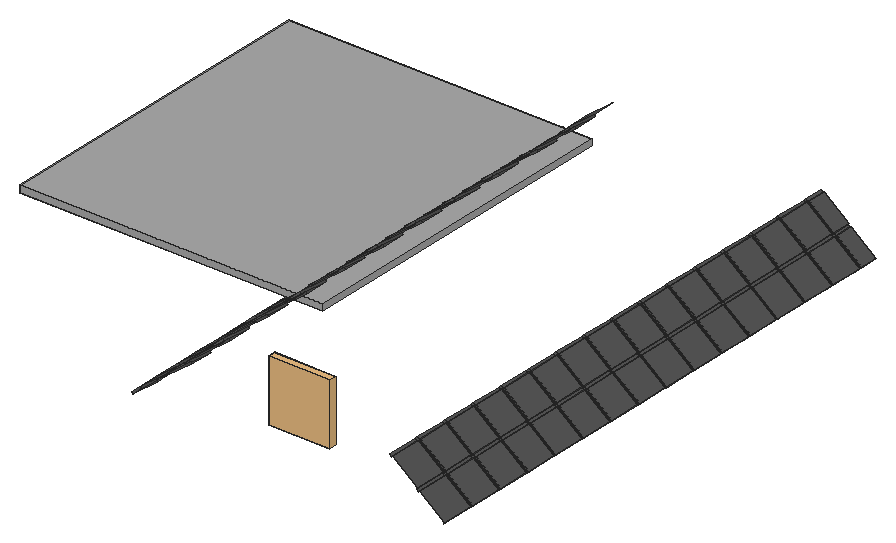
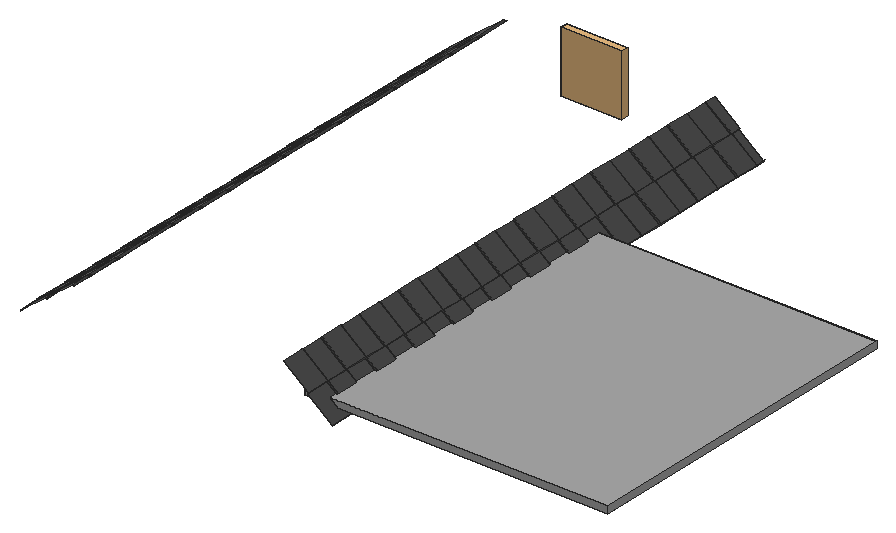
# SketchUp Ruby script. Lengths in inches.
U = 1.inch
M = Sketchup.active_model
def pt(a) = Geom::Point3d.new(a.map { |v| v * U })
def face(e, loops, mat)
  f = e.add_face(loops[0].map { |a| pt(a) })
  loops[1..].each { |l| e.add_face(l.map { |a| pt(a) }).erase! }
  f.material = f.back_material = mat if mat
  f
end
# faces: each face lists its corners as indices into pts; further lists are holes
def faces(e, pts, list, mat = nil) = list.each { |f| face(e, (f[0].is_a?(Array) ? f : [f]).map { |l| l.map { |i| pts[i] } }, mat) }
# xy, xz, yz: faces in a plane at the given z, y or x. An outline is a flat list of corners, or four numbers for a rectangle; further outlines are holes
def ring(l) = l.size == 4 ? [[l[0], l[1]], [l[2], l[1]], [l[2], l[3]], [l[0], l[3]]] : l.each_slice(2).to_a
def flat(e, list, mat, &to3) = list.each { |f| face(e, (f[0].is_a?(Array) ? f : [f]).map { |l| ring(l).map { |u, v| to3.(u, v) } }, mat) }
def xy(e, z, list, mat = nil) = flat(e, list, mat) { |x, y| [x, y, z] }
def xz(e, y, list, mat = nil) = flat(e, list, mat) { |x, z| [x, y, z] }
def yz(e, x, list, mat = nil) = flat(e, list, mat) { |y, z| [x, y, z] }
def lines(e, pts, list) = list.each { |a, b| e.add_line(pt(pts[a]), pt(pts[b])) }
# prism: a flat outline (further loops are holes) pulled along v
def prism(e, loops, v, mat = nil)
  f = face(e, loops, mat); d = Geom::Vector3d.new(v.map { |x| x * U })
  f.pushpull(f.normal.samedirection?(d) ? d.length : -d.length)
end
def box(e, o, s, mat = nil) = prism(e, [[o, [o[0] + s[0], o[1], o[2]], [o[0] + s[0], o[1] + s[1], o[2]], [o[0], o[1] + s[1], o[2]]]], [0, 0, s[2]], mat)
def at(x, y, z, deg = 0) = Geom::Transformation.translation(pt([x, y, z])) * Geom::Transformation.rotation(ORIGIN, Z_AXIS, deg.degrees)
def axes(o, x, y, z) = Geom::Transformation.new([*x, 0, *y, 0, *z, 0, *pt(o).to_a, 1])
def part(name) = M.definitions.add(name)
# library, detail: a bought-in or finely detailed component or shape, given as its bounding box
def library(name, o, s) = part(name).tap { |d| box(d.entities, o, s) }
def detail(e, o, s) = box(e.add_group.entities, o, s)
def put(e, d, t, mat = nil) = e.add_instance(d, t).tap { |i| i.material = mat if mat }
def group(e, t, mat = nil) = e.add_group.tap { |g| g.transformation = t; g.material = mat if mat }.entities
root = M.entities
M.materials.add("[Color M03]").color = [170, 170, 170]
M.materials.add("[Color M05]").color = [114, 114, 114]
M.materials.add("[Color M06]").color = [86, 86, 86]
c1 = library("Group\#78",[0,-0.5,0],[45.98,5.5,45.98])
xz(root,145.1875,[[263.93,349.38,282.83,364.17,282.34,364.8,282.03,365.19,263.13,350.4,263.4375,350.01],[282.83,364.17,282.34,364.8,282.03,365.19,300.93,379.98,301.24,379.59,301.73,378.96]],"[Color M06]")
xz(root,161.375,[[497.33,344.21,478.43,359.01,479.05,359.79,497.95,345],[476.86,360.24,457.95,375.03,458.57,375.82,477.47,361.03]],"[Color M06]")
xz(root,163.1875,[[263.93,349.38,263.4375,350.01,263.13,350.4,282.03,365.19,282.34,364.8,282.83,364.17],[282.83,364.17,301.73,378.96,301.24,379.59,300.93,379.98,282.03,365.19,282.34,364.8]],"[Color M06]")
xz(root,163.375,[[497.33,344.21,497.95,345,479.05,359.79,478.43,359.01],[476.86,360.24,477.47,361.03,458.57,375.82,457.95,375.03]],"[Color M06]")
xz(root,181.1875,[[263.93,349.38,282.83,364.17,282.34,364.8,282.03,365.19,263.13,350.4,263.4375,350.01],[282.83,364.17,282.34,364.8,282.03,365.19,300.93,379.98,301.24,379.59,301.73,378.96]],"[Color M06]")
xz(root,187.375,[[497.33,344.21,478.43,359.01,479.05,359.79,497.95,345],[476.86,360.24,457.95,375.03,458.57,375.82,477.47,361.03]],"[Color M06]")
xz(root,189.375,[[497.33,344.21,497.95,345,479.05,359.79,478.43,359.01],[476.86,360.24,477.47,361.03,458.57,375.82,457.95,375.03]],"[Color M06]")
xz(root,199.1875,[[263.93,349.38,263.4375,350.01,263.13,350.4,282.03,365.19,282.34,364.8,282.83,364.17],[282.83,364.17,301.73,378.96,301.24,379.59,300.93,379.98,282.03,365.19,282.34,364.8]],"[Color M06]")
xz(root,213.375,[[497.33,344.21,478.43,359.01,479.05,359.79,497.95,345],[476.86,360.24,457.95,375.03,458.57,375.82,477.47,361.03]],"[Color M06]")
xz(root,215.375,[[497.33,344.21,497.95,345,479.05,359.79,478.43,359.01],[476.86,360.24,477.47,361.03,458.57,375.82,457.95,375.03]],"[Color M06]")
xz(root,217.1875,[[263.93,349.38,282.83,364.17,282.34,364.8,282.03,365.19,263.13,350.4,263.4375,350.01],[282.83,364.17,282.34,364.8,282.03,365.19,300.93,379.98,301.24,379.59,301.73,378.96]],"[Color M06]")
xz(root,235.1875,[[263.93,349.38,263.4375,350.01,263.13,350.4,282.03,365.19,282.34,364.8,282.83,364.17],[282.83,364.17,301.73,378.96,301.24,379.59,300.93,379.98,282.03,365.19,282.34,364.8]],"[Color M06]")
xz(root,239.375,[[497.33,344.21,478.43,359.01,479.05,359.79,497.95,345],[476.86,360.24,457.95,375.03,458.57,375.82,477.47,361.03]],"[Color M06]")
xz(root,241.375,[[497.33,344.21,497.95,345,479.05,359.79,478.43,359.01],[476.86,360.24,477.47,361.03,458.57,375.82,457.95,375.03]],"[Color M06]")
xz(root,253.1875,[[263.93,349.38,282.83,364.17,282.34,364.8,282.03,365.19,263.13,350.4,263.4375,350.01],[282.83,364.17,282.34,364.8,282.03,365.19,300.93,379.98,301.24,379.59,301.73,378.96]],"[Color M06]")
xz(root,265.375,[[497.33,344.21,478.43,359.01,479.05,359.79,497.95,345],[476.86,360.24,457.95,375.03,458.57,375.82,477.47,361.03]],"[Color M06]")
xz(root,267.375,[[497.33,344.21,497.95,345,479.05,359.79,478.43,359.01],[476.86,360.24,477.47,361.03,458.57,375.82,457.95,375.03]],"[Color M06]")
xz(root,271.1875,[[263.93,349.38,263.4375,350.01,263.13,350.4,282.03,365.19,282.34,364.8,282.83,364.17],[282.83,364.17,301.73,378.96,301.24,379.59,300.93,379.98,282.03,365.19,282.34,364.8]],"[Color M06]")
xz(root,289.1875,[[263.93,349.38,282.83,364.17,282.34,364.8,282.03,365.19,263.13,350.4,263.4375,350.01],[282.83,364.17,282.34,364.8,282.03,365.19,300.93,379.98,301.24,379.59,301.73,378.96]],"[Color M06]")
xz(root,291.375,[[497.33,344.21,478.43,359.01,479.05,359.79,497.95,345],[476.86,360.24,457.95,375.03,458.57,375.82,477.47,361.03]],"[Color M06]")
xz(root,293.375,[[497.33,344.21,497.95,345,479.05,359.79,478.43,359.01],[476.86,360.24,477.47,361.03,458.57,375.82,457.95,375.03]],"[Color M06]")
xz(root,307.1875,[[263.93,349.38,263.4375,350.01,263.13,350.4,282.03,365.19,282.34,364.8,282.83,364.17],[282.83,364.17,301.73,378.96,301.24,379.59,300.93,379.98,282.03,365.19,282.34,364.8]],"[Color M06]")
xz(root,317.375,[[497.33,344.21,478.43,359.01,479.05,359.79,497.95,345],[476.86,360.24,457.95,375.03,458.57,375.82,477.47,361.03]],"[Color M06]")
xz(root,319.375,[[497.33,344.21,497.95,345,479.05,359.79,478.43,359.01],[476.86,360.24,477.47,361.03,458.57,375.82,457.95,375.03]],"[Color M06]")
xz(root,325.1875,[[263.93,349.38,282.83,364.17,282.34,364.8,282.03,365.19,263.13,350.4,263.4375,350.01],[282.83,364.17,282.34,364.8,282.03,365.19,300.93,379.98,301.73,378.96]],"[Color M06]")
xz(root,343.1875,[[263.93,349.38,263.4375,350.01,263.13,350.4,282.03,365.19,282.34,364.8,282.83,364.17],[282.83,364.17,301.73,378.96,300.93,379.98,282.03,365.19,282.34,364.8]],"[Color M06]")
xz(root,343.375,[[497.33,344.21,478.43,359.01,479.05,359.79,497.95,345],[476.86,360.24,457.95,375.03,458.57,375.82,477.47,361.03]],"[Color M06]")
xz(root,345.375,[[497.33,344.21,497.95,345,479.05,359.79,478.43,359.01],[476.86,360.24,477.47,361.03,458.57,375.82,457.95,375.03]],"[Color M06]")
xz(root,361.1875,[[263.93,349.38,282.83,364.17,282.34,364.8,282.03,365.19,263.13,350.4,263.4375,350.01],[282.83,364.17,282.34,364.8,282.03,365.19,300.93,379.98,301.24,379.59,301.73,378.96]],"[Color M06]")
xz(root,369.375,[[497.33,344.21,478.43,359.01,479.05,359.79,497.95,345],[476.86,360.24,457.95,375.03,458.57,375.82,477.47,361.03]],"[Color M06]")
xz(root,371.375,[[497.33,344.21,497.95,345,479.05,359.79,478.43,359.01],[476.86,360.24,477.47,361.03,458.57,375.82,457.95,375.03]],"[Color M06]")
xz(root,379.1875,[[263.93,349.38,263.4375,350.01,263.13,350.4,282.03,365.19,282.34,364.8,282.83,364.17],[282.83,364.17,301.73,378.96,301.24,379.59,300.93,379.98,282.03,365.19,282.34,364.8]],"[Color M06]")
xz(root,395.375,[[497.33,344.21,478.43,359.01,479.05,359.79,497.95,345],[476.86,360.24,457.95,375.03,458.57,375.82,477.47,361.03]],"[Color M06]")
xz(root,397.1875,[[263.93,349.38,282.83,364.17,282.34,364.8,282.03,365.19,263.13,350.4,263.4375,350.01],[282.83,364.17,282.34,364.8,282.03,365.19,300.93,379.98,301.24,379.59,301.73,378.96]],"[Color M06]")
xz(root,397.375,[[497.33,344.21,497.95,345,479.05,359.79,478.43,359.01],[476.86,360.24,477.47,361.03,458.57,375.82,457.95,375.03]],"[Color M06]")
xz(root,415.1875,[[263.93,349.38,263.4375,350.01,263.13,350.4,282.03,365.19,282.34,364.8,282.83,364.17],[282.83,364.17,301.73,378.96,301.24,379.59,300.93,379.98,282.03,365.19,282.34,364.8]],"[Color M06]")
xz(root,421.375,[[497.33,344.21,478.43,359.01,479.05,359.79,497.95,345],[476.86,360.24,457.95,375.03,458.57,375.82,477.47,361.03]],"[Color M06]")
xz(root,423.375,[[497.33,344.21,497.95,345,479.05,359.79,478.43,359.01],[476.86,360.24,477.47,361.03,458.57,375.82,457.95,375.03]],"[Color M06]")
xz(root,433.1875,[[263.93,349.38,282.83,364.17,282.34,364.8,282.03,365.19,263.13,350.4,263.4375,350.01],[282.83,364.17,282.34,364.8,282.03,365.19,300.93,379.98,301.24,379.59,301.73,378.96]],"[Color M06]")
xz(root,447.375,[[497.33,344.21,478.43,359.01,479.05,359.79,497.95,345],[476.86,360.24,457.95,375.03,458.57,375.82,477.47,361.03]],"[Color M06]")
xz(root,449.375,[[497.33,344.21,497.95,345,479.05,359.79,478.43,359.01],[476.86,360.24,477.47,361.03,458.57,375.82,457.95,375.03]],"[Color M06]")
xz(root,451.1875,[[263.93,349.38,263.4375,350.01,263.13,350.4,282.03,365.19,282.34,364.8,282.83,364.17],[282.83,364.17,301.73,378.96,301.24,379.59,300.93,379.98,282.03,365.19,282.34,364.8]],"[Color M06]")
xz(root,469.1875,[[263.93,349.38,282.83,364.17,282.34,364.8,282.03,365.19,263.13,350.4,263.4375,350.01],[282.83,364.17,282.34,364.8,282.03,365.19,300.93,379.98,301.24,379.59,301.73,378.96]],"[Color M06]")
xz(root,473.375,[[497.33,344.21,478.43,359.01,479.05,359.79,497.95,345],[476.86,360.24,457.95,375.03,458.57,375.82,477.47,361.03]],"[Color M06]")
xz(root,475.375,[[497.33,344.21,497.95,345,479.05,359.79,478.43,359.01],[476.86,360.24,477.47,361.03,458.57,375.82,457.95,375.03]],"[Color M06]")
xz(root,487.1875,[[263.93,349.38,263.4375,350.01,263.13,350.4,282.03,365.19,282.34,364.8,282.83,364.17],[282.83,364.17,301.73,378.96,301.24,379.59,300.93,379.98,282.03,365.19,282.34,364.8]],"[Color M06]")
xz(root,499.375,[[497.33,344.21,478.43,359.01,479.05,359.79,497.95,345],[476.86,360.24,457.95,375.03,458.57,375.82,477.47,361.03]],"[Color M06]")
xz(root,501.375,[[497.33,344.21,497.95,345,479.05,359.79,478.43,359.01],[476.86,360.24,477.47,361.03,458.57,375.82,457.95,375.03]],"[Color M06]")
xz(root,505.1875,[[263.93,349.38,282.83,364.17,282.34,364.8,263.4375,350.01],[282.83,364.17,282.34,364.8,282.03,365.19,300.93,379.98,301.24,379.59,301.73,378.96]],"[Color M06]")
xz(root,523.1875,[[263.93,349.38,263.4375,350.01,282.34,364.8,282.83,364.17],[282.83,364.17,301.73,378.96,301.24,379.59,300.93,379.98,300.88,380.04,281.98,365.25,282.34,364.8]],"[Color M06]")
xz(root,525.375,[[497.33,344.21,478.43,359.01,479.05,359.79,497.95,345],[476.86,360.24,457.95,375.03,458.57,375.82,477.47,361.03]],"[Color M06]")
xz(root,527.375,[[497.33,344.21,497.95,345,479.05,359.79,478.43,359.01],[476.86,360.24,477.47,361.03,458.57,375.82,457.95,375.03]],"[Color M06]")
p = [[497.33,137.375,344.21],[497.33,161.375,344.21],[497.95,161.375,345],[497.95,137.375,345],[497.33,163.375,344.21],[478.43,163.375,359.01],
  [478.43,161.375,359.01],[497.33,187.375,344.21],[497.95,187.375,345],[497.95,163.375,345],[497.33,189.375,344.21],[478.43,189.375,359.01],
  [478.43,187.375,359.01],[497.33,213.375,344.21],[497.95,213.375,345],[497.95,189.375,345],[497.33,215.375,344.21],[478.43,215.375,359.01],
  [478.43,213.375,359.01],[497.33,239.375,344.21],[497.95,239.375,345],[497.95,215.375,345],[497.33,241.375,344.21],[478.43,241.375,359.01],
  [478.43,239.375,359.01],[497.33,265.375,344.21],[497.95,265.375,345],[497.95,241.375,345],[497.33,267.375,344.21],[478.43,267.375,359.01],
  [478.43,265.375,359.01],[497.33,291.375,344.21],[497.95,291.375,345],[497.95,267.375,345],[497.33,293.375,344.21],[478.43,293.375,359.01],
  [478.43,291.375,359.01],[497.33,317.375,344.21],[497.95,317.375,345],[497.95,293.375,345],[497.33,319.375,344.21],[478.43,319.375,359.01],
  [478.43,317.375,359.01],[497.33,343.375,344.21],[497.95,343.375,345],[497.95,319.375,345],[497.33,345.375,344.21],[478.43,345.375,359.01],
  [478.43,343.375,359.01],[497.33,369.375,344.21],[497.95,369.375,345],[497.95,345.375,345],[497.33,371.375,344.21],[478.43,371.375,359.01],
  [478.43,369.375,359.01],[497.33,395.375,344.21],[497.95,395.375,345],[497.95,371.375,345],[497.33,397.375,344.21],[478.43,397.375,359.01],
  [478.43,395.375,359.01],[497.33,421.375,344.21],[497.95,421.375,345],[497.95,397.375,345],[497.33,423.375,344.21],[478.43,423.375,359.01],
  [478.43,421.375,359.01],[497.33,447.375,344.21],[497.95,447.375,345],[497.95,423.375,345],[497.33,449.375,344.21],[478.43,449.375,359.01],
  [478.43,447.375,359.01],[497.33,473.375,344.21],[497.95,473.375,345],[497.95,449.375,345],[497.33,475.375,344.21],[478.43,475.375,359.01],
  [478.43,473.375,359.01],[497.33,499.375,344.21],[497.95,499.375,345],[497.95,475.375,345],[497.33,501.375,344.21],[478.43,501.375,359.01],
  [478.43,499.375,359.01],[497.33,525.375,344.21],[497.95,525.375,345],[497.95,501.375,345],[497.33,527.375,344.21],[478.43,527.375,359.01],
  [478.43,525.375,359.01],[497.33,541.1875,344.21],[497.95,541.1875,345],[497.95,527.375,345],[479.05,161.375,359.79],[479.05,137.375,359.79],
  [479.05,187.375,359.79],[479.05,163.375,359.79],[479.05,213.375,359.79],[479.05,189.375,359.79],[479.05,239.375,359.79],[479.05,215.375,359.79],
  [479.05,265.375,359.79],[479.05,241.375,359.79],[479.05,291.375,359.79],[479.05,267.375,359.79],[479.05,317.375,359.79],[479.05,293.375,359.79],
  [479.05,343.375,359.79],[479.05,319.375,359.79],[479.05,369.375,359.79],[479.05,345.375,359.79],[479.05,395.375,359.79],[479.05,371.375,359.79],
  [479.05,421.375,359.79],[479.05,397.375,359.79],[479.05,447.375,359.79],[479.05,423.375,359.79],[479.05,473.375,359.79],[479.05,449.375,359.79],
  [479.05,499.375,359.79],[479.05,475.375,359.79],[479.05,525.375,359.79],[479.05,501.375,359.79],[479.05,541.1875,359.79],[479.05,527.375,359.79],
  [263.93,137.375,349.38],[263.93,145.1875,349.38],[263.4375,145.1875,350.01],[263.13,145.1875,350.4],[263.13,137.375,350.4],[282.83,145.1875,364.17],
  [282.83,137.375,364.17],[263.93,163.1875,349.38],[263.13,163.1875,350.4],[263.4375,163.1875,350.01],[263.93,181.1875,349.38],[263.4375,181.1875,350.01],
  [263.13,181.1875,350.4],[282.83,181.1875,364.17],[282.83,163.1875,364.17],[263.93,199.1875,349.38],[263.13,199.1875,350.4],[263.4375,199.1875,350.01],
  [263.93,217.1875,349.38],[263.4375,217.1875,350.01],[263.13,217.1875,350.4],[282.83,217.1875,364.17],[282.83,199.1875,364.17],[263.93,235.1875,349.38],
  [263.13,235.1875,350.4],[263.4375,235.1875,350.01],[263.93,253.1875,349.38],[263.4375,253.1875,350.01],[263.13,253.1875,350.4],[282.83,253.1875,364.17],
  [282.83,235.1875,364.17],[263.93,271.1875,349.38],[263.13,271.1875,350.4],[263.4375,271.1875,350.01],[263.93,289.1875,349.38],[263.4375,289.1875,350.01],
  [263.13,289.1875,350.4],[282.83,289.1875,364.17],[282.83,271.1875,364.17],[263.93,307.1875,349.38],[263.13,307.1875,350.4],[263.4375,307.1875,350.01],
  [263.93,325.1875,349.38],[263.4375,325.1875,350.01],[263.13,325.1875,350.4],[282.83,325.1875,364.17],[282.83,307.1875,364.17],[263.93,343.1875,349.38],
  [263.13,343.1875,350.4],[263.4375,343.1875,350.01],[263.93,361.1875,349.38],[263.4375,361.1875,350.01],[263.13,361.1875,350.4],[282.83,361.1875,364.17],
  [282.83,343.1875,364.17],[263.93,379.1875,349.38],[263.13,379.1875,350.4],[263.4375,379.1875,350.01],[263.93,397.1875,349.38],[263.4375,397.1875,350.01],
  [263.13,397.1875,350.4],[282.83,397.1875,364.17],[282.83,379.1875,364.17],[263.93,415.1875,349.38],[263.13,415.1875,350.4],[263.4375,415.1875,350.01],
  [263.93,433.1875,349.38],[263.4375,433.1875,350.01],[263.13,433.1875,350.4],[282.83,433.1875,364.17],[282.83,415.1875,364.17],[263.93,451.1875,349.38],
  [263.13,451.1875,350.4],[263.4375,451.1875,350.01],[263.93,469.1875,349.38],[263.4375,469.1875,350.01],[263.13,469.1875,350.4],[282.83,469.1875,364.17],
  [282.83,451.1875,364.17],[263.93,487.1875,349.38],[263.13,487.1875,350.4],[263.4375,487.1875,350.01],[263.93,505.1875,349.38],[263.4375,505.1875,350.01],
  [263.13,505.1875,350.4],[282.83,505.1875,364.17],[282.83,487.1875,364.17],[263.93,523.1875,349.38],[263.4375,523.1875,350.01],[263.93,541.1875,349.38],
  [263.08,541.1875,350.46],[263.08,523.1875,350.46],[282.83,541.1875,364.17],[282.83,523.1875,364.17],[282.34,523.1875,364.8],[282.34,505.1875,364.8],
  [282.03,163.1875,365.19],[282.03,145.1875,365.19],[282.03,199.1875,365.19],[282.03,181.1875,365.19],[282.03,235.1875,365.19],[282.03,217.1875,365.19],
  [282.03,271.1875,365.19],[282.03,253.1875,365.19],[282.03,307.1875,365.19],[282.03,289.1875,365.19],[282.03,343.1875,365.19],[282.03,325.1875,365.19],
  [282.03,379.1875,365.19],[282.03,361.1875,365.19],[282.03,415.1875,365.19],[282.03,397.1875,365.19],[282.03,451.1875,365.19],[282.03,433.1875,365.19],
  [282.03,487.1875,365.19],[282.03,469.1875,365.19],[476.86,161.375,360.24],[476.86,137.375,360.24],[478.43,137.375,359.01],[476.86,163.375,360.24],
  [476.86,187.375,360.24],[476.86,189.375,360.24],[476.86,213.375,360.24],[476.86,215.375,360.24],[476.86,239.375,360.24],[476.86,241.375,360.24],
  [476.86,265.375,360.24],[476.86,267.375,360.24],[476.86,291.375,360.24],[476.86,293.375,360.24],[476.86,317.375,360.24],[476.86,319.375,360.24],
  [476.86,343.375,360.24],[476.86,345.375,360.24],[476.86,369.375,360.24],[476.86,371.375,360.24],[476.86,395.375,360.24],[476.86,397.375,360.24],
  [476.86,421.375,360.24],[476.86,423.375,360.24],[476.86,447.375,360.24],[476.86,449.375,360.24],[476.86,473.375,360.24],[476.86,475.375,360.24],
  [476.86,499.375,360.24],[476.86,501.375,360.24],[476.86,525.375,360.24],[476.86,527.375,360.24],[478.43,541.1875,359.01],[476.86,541.1875,360.24],
  [477.47,161.375,361.03],[477.47,137.375,361.03],[457.95,163.375,375.03],[457.95,161.375,375.03],[477.47,187.375,361.03],[477.47,163.375,361.03],
  [457.95,189.375,375.03],[457.95,187.375,375.03],[477.47,213.375,361.03],[477.47,189.375,361.03],[457.95,215.375,375.03],[457.95,213.375,375.03],
  [477.47,239.375,361.03],[477.47,215.375,361.03],[457.95,241.375,375.03],[457.95,239.375,375.03],[477.47,265.375,361.03],[477.47,241.375,361.03],
  [457.95,267.375,375.03],[457.95,265.375,375.03],[477.47,291.375,361.03],[477.47,267.375,361.03],[457.95,293.375,375.03],[457.95,291.375,375.03],
  [477.47,317.375,361.03],[477.47,293.375,361.03],[457.95,319.375,375.03],[457.95,317.375,375.03],[477.47,343.375,361.03],[477.47,319.375,361.03],
  [457.95,345.375,375.03],[457.95,343.375,375.03],[477.47,369.375,361.03],[477.47,345.375,361.03],[457.95,371.375,375.03],[457.95,369.375,375.03],
  [477.47,395.375,361.03],[477.47,371.375,361.03],[457.95,397.375,375.03],[457.95,395.375,375.03],[477.47,421.375,361.03],[477.47,397.375,361.03],
  [457.95,423.375,375.03],[457.95,421.375,375.03],[477.47,447.375,361.03],[477.47,423.375,361.03],[457.95,449.375,375.03],[457.95,447.375,375.03],
  [477.47,473.375,361.03],[477.47,449.375,361.03],[457.95,475.375,375.03],[457.95,473.375,375.03],[477.47,499.375,361.03],[477.47,475.375,361.03],
  [457.95,501.375,375.03],[457.95,499.375,375.03],[477.47,525.375,361.03],[477.47,501.375,361.03],[457.95,527.375,375.03],[457.95,525.375,375.03],
  [477.47,541.1875,361.03],[477.47,527.375,361.03],[458.57,161.375,375.82],[458.57,137.375,375.82],[458.57,187.375,375.82],[458.57,163.375,375.82],
  [458.57,213.375,375.82],[458.57,189.375,375.82],[458.57,239.375,375.82],[458.57,215.375,375.82],[458.57,265.375,375.82],[458.57,241.375,375.82],
  [458.57,291.375,375.82],[458.57,267.375,375.82],[458.57,317.375,375.82],[458.57,293.375,375.82],[458.57,343.375,375.82],[458.57,319.375,375.82],
  [458.57,369.375,375.82],[458.57,345.375,375.82],[458.57,395.375,375.82],[458.57,371.375,375.82],[458.57,421.375,375.82],[458.57,397.375,375.82],
  [458.57,447.375,375.82],[458.57,423.375,375.82],[458.57,473.375,375.82],[458.57,449.375,375.82],[458.57,499.375,375.82],[458.57,475.375,375.82],
  [458.57,525.375,375.82],[458.57,501.375,375.82],[458.57,541.1875,375.82],[458.57,527.375,375.82],[282.03,137.375,365.19],[282.34,145.1875,364.8],
  [282.34,163.1875,364.8],[301.73,163.1875,378.96],[301.73,145.1875,378.96],[282.34,181.1875,364.8],[282.34,199.1875,364.8],[301.73,199.1875,378.96],
  [301.73,181.1875,378.96],[282.34,217.1875,364.8],[282.34,235.1875,364.8],[301.73,235.1875,378.96],[301.73,217.1875,378.96],[282.34,253.1875,364.8],
  [282.34,271.1875,364.8],[301.73,271.1875,378.96],[301.73,253.1875,378.96],[282.34,289.1875,364.8],[282.34,307.1875,364.8],[301.73,307.1875,378.96],
  [301.73,289.1875,378.96],[282.34,325.1875,364.8],[282.34,343.1875,364.8],[301.73,343.1875,378.96],[301.73,325.1875,378.96],[282.34,361.1875,364.8],
  [282.34,379.1875,364.8],[301.73,379.1875,378.96],[301.73,361.1875,378.96],[282.34,397.1875,364.8],[282.34,415.1875,364.8],[301.73,415.1875,378.96],
  [301.73,397.1875,378.96],[282.34,433.1875,364.8],[282.34,451.1875,364.8],[301.73,451.1875,378.96],[301.73,433.1875,378.96],[282.34,469.1875,364.8],
  [282.34,487.1875,364.8],[301.73,487.1875,378.96],[301.73,469.1875,378.96],[282.03,505.1875,365.19],[301.73,523.1875,378.96],[301.73,505.1875,378.96],
  [281.98,523.1875,365.25],[281.98,541.1875,365.25],[300.93,145.1875,379.98],[300.93,137.375,379.98],[300.93,181.1875,379.98],[300.93,163.1875,379.98],
  [300.93,217.1875,379.98],[300.93,199.1875,379.98],[300.93,253.1875,379.98],[300.93,235.1875,379.98],[300.93,289.1875,379.98],[300.93,271.1875,379.98],
  [300.93,325.1875,379.98],[300.93,307.1875,379.98],[300.93,361.1875,379.98],[300.93,343.1875,379.98],[300.93,397.1875,379.98],[300.93,379.1875,379.98],
  [300.93,433.1875,379.98],[300.93,415.1875,379.98],[300.93,469.1875,379.98],[300.93,451.1875,379.98],[300.93,505.1875,379.98],[300.93,487.1875,379.98],
  [300.88,541.1875,380.04],[300.88,523.1875,380.04],[456.38,161.375,376.26],[456.38,137.375,376.26],[457.95,137.375,375.03],[456.38,163.375,376.26],
  [456.38,187.375,376.26],[456.38,189.375,376.26],[456.38,213.375,376.26],[456.38,215.375,376.26],[456.38,239.375,376.26],[456.38,241.375,376.26],
  [456.38,265.375,376.26],[456.38,267.375,376.26],[456.38,291.375,376.26],[456.38,293.375,376.26],[456.38,317.375,376.26],[456.38,319.375,376.26],
  [456.38,343.375,376.26],[456.38,345.375,376.26],[456.38,369.375,376.26],[456.38,371.375,376.26],[456.38,395.375,376.26],[456.38,397.375,376.26],
  [456.38,421.375,376.26],[456.38,423.375,376.26],[456.38,447.375,376.26],[456.38,449.375,376.26],[456.38,473.375,376.26],[456.38,475.375,376.26],
  [456.38,499.375,376.26],[456.38,501.375,376.26],[456.38,525.375,376.26],[456.38,527.375,376.26],[457.95,541.1875,375.03],[456.38,541.1875,376.26]]
faces(root,p,[[0,1,2,3],[4,5,6,1],[4,7,8,9],[10,11,12,7],[10,13,14,15],[16,17,18,13],[16,19,20,21],[22,23,24,19],
  [22,25,26,27],[28,29,30,25],[28,31,32,33],[34,35,36,31],[34,37,38,39],[40,41,42,37],[40,43,44,45],[46,47,48,43],
  [46,49,50,51],[52,53,54,49],[52,55,56,57],[58,59,60,55],[58,61,62,63],[64,65,66,61],[64,67,68,69],[70,71,72,67],
  [70,73,74,75],[76,77,78,73],[76,79,80,81],[82,83,84,79],[82,85,86,87],[88,89,90,85],[88,91,92,93],[2,94,95,3],
  [8,96,97,9],[14,98,99,15],[20,100,101,21],[26,102,103,27],[32,104,105,33],[38,106,107,39],[44,108,109,45],[50,110,111,51],
  [56,112,113,57],[62,114,115,63],[68,116,117,69],[74,118,119,75],[80,120,121,81],[86,122,123,87],[92,124,125,93],[126,127,128,129,130],
  [131,127,126,132],[133,127,128,129,134,135],[133,136,137,138,134,135],[139,136,133,140],[141,136,137,138,142,143],[141,144,145,146,142,143],[147,144,141,148],[149,144,145,146,150,151],
  [149,152,153,154,150,151],[155,152,149,156],[157,152,153,154,158,159],[157,160,161,162,158,159],[163,160,157,164],[165,160,161,162,166,167],[165,168,169,170,166,167],[171,168,165,172],
  [173,168,169,170,174,175],[173,176,177,178,174,175],[179,176,173,180],[181,176,177,178,182,183],[181,184,185,186,182,183],[187,184,181,188],[189,184,185,186,190,191],[189,192,193,194,190,191],
  [195,192,189,196],[197,192,193,194,198,199],[197,200,201,202,198,199],[203,200,197,204],[205,200,201,202,206,207],[205,208,209,210,206,207],[211,208,205,212],[213,208,209,214],
  [213,215,216,217,214],[218,215,213,219],[220,214,209,221],[222,134,129,223],[224,142,138,225],[226,150,146,227],[228,158,154,229],[230,166,162,231],
  [232,174,170,233],[234,182,178,235],[236,190,186,237],[238,198,194,239],[240,206,202,241],[6,242,243,244],[6,244,95,94],[242,6,5,245],
  [12,246,245,5],[12,5,97,96],[11,247,246,12],[18,248,247,11],[18,11,99,98],[17,249,248,18],[249,17,24,250],[24,17,101,100],
  [23,251,250,24],[30,252,251,23],[30,23,103,102],[252,30,29,253],[253,29,36,254],[36,29,105,104],[254,36,35,255],[255,35,42,256],
  [42,35,107,106],[256,42,41,257],[257,41,48,258],[48,41,109,108],[47,259,258,48],[54,260,259,47],[54,47,111,110],[260,54,53,261],
  [261,53,60,262],[60,53,113,112],[59,263,262,60],[66,264,263,59],[66,59,115,114],[65,265,264,66],[265,65,72,266],[72,65,117,116],
  [266,72,71,267],[267,71,78,268],[78,71,119,118],[77,269,268,78],[84,270,269,77],[84,77,121,120],[270,84,83,271],[271,83,90,272],
  [90,83,123,122],[89,273,272,90],[274,275,273,89],[274,89,125,124],[243,242,276,277],[245,278,279,242],[245,246,280,281],[247,282,283,246],
  [247,248,284,285],[249,286,287,248],[249,250,288,289],[251,290,291,250],[251,252,292,293],[253,294,295,252],[253,254,296,297],[255,298,299,254],
  [255,256,300,301],[257,302,303,256],[257,258,304,305],[259,306,307,258],[259,260,308,309],[261,310,311,260],[261,262,312,313],[263,314,315,262],
  [263,264,316,317],[265,318,319,264],[265,266,320,321],[267,322,323,266],[267,268,324,325],[269,326,327,268],[269,270,328,329],[271,330,331,270],
  [271,272,332,333],[273,334,335,272],[273,275,336,337],[276,338,339,277],[280,340,341,281],[284,342,343,285],[288,344,345,289],[292,346,347,293],
  [296,348,349,297],[300,350,351,301],[304,352,353,305],[308,354,355,309],[312,356,357,313],[316,358,359,317],[320,360,361,321],[324,362,363,325],
  [328,364,365,329],[332,366,367,333],[336,368,369,337],[131,132,370,223,371],[131,140,372,222,223,371],[373,140,131,374],[139,140,372,222,225,375],[139,148,376,224,225,375],
  [377,148,139,378],[147,148,376,224,227,379],[147,156,380,226,227,379],[381,156,147,382],[155,156,380,226,229,383],[155,164,384,228,229,383],[385,164,155,386],[163,164,384,228,231,387],
  [163,172,388,230,231,387],[389,172,163,390],[171,172,388,230,233,391],[171,180,392,232,233,391],[393,180,171,394],[179,180,392,232,235,395],[179,188,396,234,235,395],[397,188,179,398],
  [187,188,396,234,237,399],[187,196,400,236,237,399],[401,196,187,402],[195,196,400,236,239,403],[195,204,404,238,239,403],[405,204,195,406],[203,204,404,238,241,407],[203,212,408,240,241,407],
  [409,212,203,410],[211,212,408,240,411,221],[211,219,220,221],[412,219,211,413],[218,219,220,414,415],[416,223,370,417],[418,225,222,419],[420,227,224,421],
  [422,229,226,423],[424,231,228,425],[426,233,230,427],[428,235,232,429],[430,237,234,431],[432,239,236,433],[434,241,238,435],[436,411,240,437],
  [438,415,414,439],[279,440,441,442],[279,442,339,338],[278,443,440,279],[283,444,443,278],[283,278,341,340],[282,445,444,283],[287,446,445,282],
  [287,282,343,342],[446,287,286,447],[447,286,291,448],[291,286,345,344],[448,291,290,449],[449,290,295,450],[295,290,347,346],[294,451,450,295],
  [451,294,299,452],[299,294,349,348],[298,453,452,299],[303,454,453,298],[303,298,351,350],[454,303,302,455],[307,456,455,302],[307,302,353,352],
  [306,457,456,307],[311,458,457,306],[311,306,355,354],[310,459,458,311],[459,310,315,460],[315,310,357,356],[314,461,460,315],[319,462,461,314],
  [319,314,359,358],[318,463,462,319],[463,318,323,464],[323,318,361,360],[464,323,322,465],[327,466,465,322],[327,322,363,362],[466,327,326,467],
  [467,326,331,468],[331,326,365,364],[468,331,330,469],[469,330,335,470],[335,330,367,366],[334,471,470,335],[471,334,472,473],[472,334,369,368]],"[Color M06]")
g1 = group(root,at(70.83,280.375,354),"[Color M03]")
box(g1,[-3,-3,0],[226.5,251.8125,5])
put(root,c1,at(354.34,152.08,354.21),"[Color M05]")
